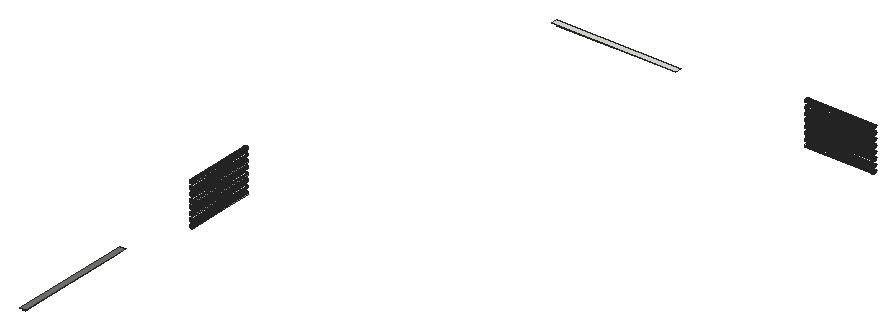
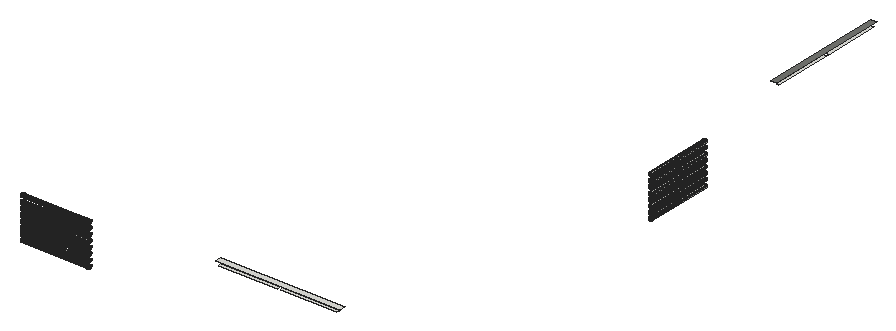
# SketchUp Ruby script. Lengths in inches.
U = 1.inch
M = Sketchup.active_model
def pt(a) = Geom::Point3d.new(a.map { |v| v * U })
def face(e, loops, mat)
  f = e.add_face(loops[0].map { |a| pt(a) })
  loops[1..].each { |l| e.add_face(l.map { |a| pt(a) }).erase! }
  f.material = f.back_material = mat if mat
  f
end
# faces: each face lists its corners as indices into pts; further lists are holes
def faces(e, pts, list, mat = nil) = list.each { |f| face(e, (f[0].is_a?(Array) ? f : [f]).map { |l| l.map { |i| pts[i] } }, mat) }
# xy, xz, yz: faces in a plane at the given z, y or x. An outline is a flat list of corners, or four numbers for a rectangle; further outlines are holes
def ring(l) = l.size == 4 ? [[l[0], l[1]], [l[2], l[1]], [l[2], l[3]], [l[0], l[3]]] : l.each_slice(2).to_a
def flat(e, list, mat, &to3) = list.each { |f| face(e, (f[0].is_a?(Array) ? f : [f]).map { |l| ring(l).map { |u, v| to3.(u, v) } }, mat) }
def xy(e, z, list, mat = nil) = flat(e, list, mat) { |x, y| [x, y, z] }
def xz(e, y, list, mat = nil) = flat(e, list, mat) { |x, z| [x, y, z] }
def yz(e, x, list, mat = nil) = flat(e, list, mat) { |y, z| [x, y, z] }
def lines(e, pts, list) = list.each { |a, b| e.add_line(pt(pts[a]), pt(pts[b])) }
# prism: a flat outline (further loops are holes) pulled along v
def prism(e, loops, v, mat = nil)
  f = face(e, loops, mat); d = Geom::Vector3d.new(v.map { |x| x * U })
  f.pushpull(f.normal.samedirection?(d) ? d.length : -d.length)
end
def box(e, o, s, mat = nil) = prism(e, [[o, [o[0] + s[0], o[1], o[2]], [o[0] + s[0], o[1] + s[1], o[2]], [o[0], o[1] + s[1], o[2]]]], [0, 0, s[2]], mat)
def at(x, y, z, deg = 0) = Geom::Transformation.translation(pt([x, y, z])) * Geom::Transformation.rotation(ORIGIN, Z_AXIS, deg.degrees)
def axes(o, x, y, z) = Geom::Transformation.new([*x, 0, *y, 0, *z, 0, *pt(o).to_a, 1])
def part(name) = M.definitions.add(name)
# library, detail: a bought-in or finely detailed component or shape, given as its bounding box
def library(name, o, s) = part(name).tap { |d| box(d.entities, o, s) }
def detail(e, o, s) = box(e.add_group.entities, o, s)
def put(e, d, t, mat = nil) = e.add_instance(d, t).tap { |i| i.material = mat if mat }
def group(e, t, mat = nil) = e.add_group.tap { |g| g.transformation = t; g.material = mat if mat }.entities
root = M.entities
M.materials.add("[Metal Seamed]").color = [118, 119, 115]
xy(root,1007.61,[[120,175.92,126,293.77],[120,299.77,126,423.61],[211.11,1458.8125,328.96,1464.8125],[334.96,1458.8125,458.8,1464.8125]])
xy(root,1013.61,[[205.11,1452.8125,464.8,1464.8125]])
xy(root,1013.61,[[120,169.92,132,429.61]],"[Metal Seamed]")
p = [[83.53,662.8,933.02],[82.57,662.8,933.14],[82.57,806.17,933.14],[83.53,806.17,933.02],[84.48,662.8,933.14],[84.48,806.17,933.14],
  [697.99,1500.33,933.14],[697.99,1501.28,933.02],[841.36,1501.28,933.02],[841.36,1500.33,933.14],[697.99,1502.24,933.14],[841.36,1502.24,933.14],
  [81.68,662.8,933.51],[81.68,806.17,933.51],[85.37,662.8,933.51],[85.37,806.17,933.51],[697.99,1499.44,933.51],[841.36,1499.44,933.51],
  [697.99,1503.13,933.51],[841.36,1503.13,933.51],[80.92,662.8,934.1],[80.92,806.17,934.1],[86.13,662.8,934.1],[86.13,806.17,934.1],
  [697.99,1498.68,934.1],[841.36,1498.68,934.1],[697.99,1503.89,934.1],[841.36,1503.89,934.1],[80.33,662.8,934.86],[80.33,806.17,934.86],
  [86.72,662.8,934.86],[86.72,806.17,934.86],[697.99,1498.09,934.86],[841.36,1498.09,934.86],[697.99,1504.48,934.86],[841.36,1504.48,934.86],
  [79.97,662.8,935.75],[79.97,806.17,935.75],[87.09,662.8,935.75],[87.09,806.17,935.75],[697.99,1497.72,935.75],[841.36,1497.72,935.75],
  [697.99,1504.85,935.75],[841.36,1504.85,935.75],[79.84,662.8,936.7],[79.84,806.17,936.7],[87.21,662.8,936.7],[87.21,806.17,936.7],
  [697.99,1497.6,936.7],[841.36,1497.6,936.7],[697.99,1504.97,936.7],[841.36,1504.97,936.7],[79.97,662.8,937.66],[79.97,806.17,937.66],
  [87.09,662.8,937.66],[87.09,806.17,937.66],[697.99,1497.72,937.66],[841.36,1497.72,937.66],[697.99,1504.85,937.66],[841.36,1504.85,937.66],
  [80.33,662.8,938.55],[80.33,806.17,938.55],[86.72,662.8,938.55],[86.72,806.17,938.55],[697.99,1498.09,938.55],[841.36,1498.09,938.55],
  [697.99,1504.48,938.55],[841.36,1504.48,938.55],[80.92,662.8,939.3125],[80.92,806.17,939.3125],[86.13,662.8,939.3125],[86.13,806.17,939.3125],
  [697.99,1498.68,939.3125],[841.36,1498.68,939.3125],[697.99,1503.89,939.3125],[841.36,1503.89,939.3125],[81.68,662.8,939.9],[81.68,806.17,939.9],
  [85.37,662.8,939.9],[85.37,806.17,939.9],[697.99,1499.44,939.9],[841.36,1499.44,939.9],[697.99,1503.13,939.9],[841.36,1503.13,939.9],
  [82.57,662.8,940.27],[82.57,806.17,940.27],[84.48,662.8,940.27],[84.48,806.17,940.27],[697.99,1500.33,940.27],[841.36,1500.33,940.27],
  [697.99,1502.24,940.27],[841.36,1502.24,940.27],[83.53,662.8,940.39],[83.53,806.17,940.39],[697.99,1501.28,940.39],[841.36,1501.28,940.39],
  [83.53,662.8,945.02],[82.57,662.8,945.14],[82.57,806.17,945.14],[83.53,806.17,945.02],[84.48,662.8,945.14],[84.48,806.17,945.14],
  [697.99,1500.33,945.14],[697.99,1501.28,945.02],[841.36,1501.28,945.02],[841.36,1500.33,945.14],[697.99,1502.24,945.14],[841.36,1502.24,945.14],
  [81.68,662.8,945.51],[81.68,806.17,945.51],[85.37,662.8,945.51],[85.37,806.17,945.51],[697.99,1499.44,945.51],[841.36,1499.44,945.51],
  [697.99,1503.13,945.51],[841.36,1503.13,945.51],[80.92,662.8,946.1],[80.92,806.17,946.1],[86.13,662.8,946.1],[86.13,806.17,946.1],
  [697.99,1498.68,946.1],[841.36,1498.68,946.1],[697.99,1503.89,946.1],[841.36,1503.89,946.1],[80.33,662.8,946.86],[80.33,806.17,946.86],
  [86.72,662.8,946.86],[86.72,806.17,946.86],[697.99,1498.09,946.86],[841.36,1498.09,946.86],[697.99,1504.48,946.86],[841.36,1504.48,946.86],
  [79.97,662.8,947.75],[79.97,806.17,947.75],[87.09,662.8,947.75],[87.09,806.17,947.75],[697.99,1497.72,947.75],[841.36,1497.72,947.75],
  [697.99,1504.85,947.75],[841.36,1504.85,947.75],[79.84,662.8,948.7],[79.84,806.17,948.7],[87.21,662.8,948.7],[87.21,806.17,948.7],
  [697.99,1497.6,948.7],[841.36,1497.6,948.7],[697.99,1504.97,948.7],[841.36,1504.97,948.7],[79.97,662.8,949.66],[79.97,806.17,949.66],
  [87.09,662.8,949.66],[87.09,806.17,949.66],[697.99,1497.72,949.66],[841.36,1497.72,949.66],[697.99,1504.85,949.66],[841.36,1504.85,949.66],
  [80.33,662.8,950.55],[80.33,806.17,950.55],[86.72,662.8,950.55],[86.72,806.17,950.55],[697.99,1498.09,950.55],[841.36,1498.09,950.55],
  [697.99,1504.48,950.55],[841.36,1504.48,950.55],[80.92,662.8,951.3125],[80.92,806.17,951.3125],[86.13,662.8,951.3125],[86.13,806.17,951.3125],
  [697.99,1498.68,951.3125],[841.36,1498.68,951.3125],[697.99,1503.89,951.3125],[841.36,1503.89,951.3125],[81.68,662.8,951.9],[81.68,806.17,951.9],
  [85.37,662.8,951.9],[85.37,806.17,951.9],[697.99,1499.44,951.9],[841.36,1499.44,951.9],[697.99,1503.13,951.9],[841.36,1503.13,951.9],
  [82.57,662.8,952.27],[82.57,806.17,952.27],[84.48,662.8,952.27],[84.48,806.17,952.27],[697.99,1500.33,952.27],[841.36,1500.33,952.27],
  [697.99,1502.24,952.27],[841.36,1502.24,952.27],[83.53,662.8,952.39],[83.53,806.17,952.39],[697.99,1501.28,952.39],[841.36,1501.28,952.39],
  [83.53,662.8,957.02],[82.57,662.8,957.14],[82.57,806.17,957.14],[83.53,806.17,957.02],[84.48,662.8,957.14],[84.48,806.17,957.14],
  [697.99,1500.33,957.14],[697.99,1501.28,957.02],[841.36,1501.28,957.02],[841.36,1500.33,957.14],[697.99,1502.24,957.14],[841.36,1502.24,957.14],
  [81.68,662.8,957.51],[81.68,806.17,957.51],[85.37,662.8,957.51],[85.37,806.17,957.51],[697.99,1499.44,957.51],[841.36,1499.44,957.51],
  [697.99,1503.13,957.51],[841.36,1503.13,957.51],[80.92,662.8,958.1],[80.92,806.17,958.1],[86.13,662.8,958.1],[86.13,806.17,958.1],
  [697.99,1498.68,958.1],[841.36,1498.68,958.1],[697.99,1503.89,958.1],[841.36,1503.89,958.1],[80.33,662.8,958.86],[80.33,806.17,958.86],
  [86.72,662.8,958.86],[86.72,806.17,958.86],[697.99,1498.09,958.86],[841.36,1498.09,958.86],[697.99,1504.48,958.86],[841.36,1504.48,958.86],
  [79.97,662.8,959.75],[79.97,806.17,959.75],[87.09,662.8,959.75],[87.09,806.17,959.75],[697.99,1497.72,959.75],[841.36,1497.72,959.75],
  [697.99,1504.85,959.75],[841.36,1504.85,959.75],[79.84,662.8,960.7],[79.84,806.17,960.7],[87.21,662.8,960.7],[87.21,806.17,960.7],
  [697.99,1497.6,960.7],[841.36,1497.6,960.7],[697.99,1504.97,960.7],[841.36,1504.97,960.7],[79.97,662.8,961.66],[79.97,806.17,961.66],
  [87.09,662.8,961.66],[87.09,806.17,961.66],[697.99,1497.72,961.66],[841.36,1497.72,961.66],[697.99,1504.85,961.66],[841.36,1504.85,961.66],
  [80.33,662.8,962.55],[80.33,806.17,962.55],[86.72,662.8,962.55],[86.72,806.17,962.55],[697.99,1498.09,962.55],[841.36,1498.09,962.55],
  [697.99,1504.48,962.55],[841.36,1504.48,962.55],[80.92,662.8,963.3125],[80.92,806.17,963.3125],[86.13,662.8,963.3125],[86.13,806.17,963.3125],
  [697.99,1498.68,963.3125],[841.36,1498.68,963.3125],[697.99,1503.89,963.3125],[841.36,1503.89,963.3125],[81.68,662.8,963.9],[81.68,806.17,963.9],
  [85.37,662.8,963.9],[85.37,806.17,963.9],[697.99,1499.44,963.9],[841.36,1499.44,963.9],[697.99,1503.13,963.9],[841.36,1503.13,963.9],
  [82.57,662.8,964.27],[82.57,806.17,964.27],[84.48,662.8,964.27],[84.48,806.17,964.27],[697.99,1500.33,964.27],[841.36,1500.33,964.27],
  [697.99,1502.24,964.27],[841.36,1502.24,964.27],[83.53,662.8,964.39],[83.53,806.17,964.39],[697.99,1501.28,964.39],[841.36,1501.28,964.39],
  [83.53,662.8,969.02],[82.57,662.8,969.14],[82.57,806.17,969.14],[83.53,806.17,969.02],[84.48,662.8,969.14],[84.48,806.17,969.14],
  [697.99,1500.33,969.14],[697.99,1501.28,969.02],[841.36,1501.28,969.02],[841.36,1500.33,969.14],[697.99,1502.24,969.14],[841.36,1502.24,969.14],
  [81.68,662.8,969.51],[81.68,806.17,969.51],[85.37,662.8,969.51],[85.37,806.17,969.51],[697.99,1499.44,969.51],[841.36,1499.44,969.51],
  [697.99,1503.13,969.51],[841.36,1503.13,969.51],[80.92,662.8,970.1],[80.92,806.17,970.1],[86.13,662.8,970.1],[86.13,806.17,970.1],
  [697.99,1498.68,970.1],[841.36,1498.68,970.1],[697.99,1503.89,970.1],[841.36,1503.89,970.1],[80.33,662.8,970.86],[80.33,806.17,970.86],
  [86.72,662.8,970.86],[86.72,806.17,970.86],[697.99,1498.09,970.86],[841.36,1498.09,970.86],[697.99,1504.48,970.86],[841.36,1504.48,970.86],
  [79.97,662.8,971.75],[79.97,806.17,971.75],[87.09,662.8,971.75],[87.09,806.17,971.75],[697.99,1497.72,971.75],[841.36,1497.72,971.75],
  [697.99,1504.85,971.75],[841.36,1504.85,971.75],[79.84,662.8,972.7],[79.84,806.17,972.7],[87.21,662.8,972.7],[87.21,806.17,972.7],
  [697.99,1497.6,972.7],[841.36,1497.6,972.7],[697.99,1504.97,972.7],[841.36,1504.97,972.7],[79.97,662.8,973.66],[79.97,806.17,973.66],
  [87.09,662.8,973.66],[87.09,806.17,973.66],[697.99,1497.72,973.66],[841.36,1497.72,973.66],[697.99,1504.85,973.66],[841.36,1504.85,973.66],
  [80.33,662.8,974.55],[80.33,806.17,974.55],[86.72,662.8,974.55],[86.72,806.17,974.55],[697.99,1498.09,974.55],[841.36,1498.09,974.55],
  [697.99,1504.48,974.55],[841.36,1504.48,974.55],[80.92,662.8,975.3125],[80.92,806.17,975.3125],[86.13,662.8,975.3125],[86.13,806.17,975.3125],
  [697.99,1498.68,975.3125],[841.36,1498.68,975.3125],[697.99,1503.89,975.3125],[841.36,1503.89,975.3125],[81.68,662.8,975.9],[81.68,806.17,975.9],
  [85.37,662.8,975.9],[85.37,806.17,975.9],[697.99,1499.44,975.9],[841.36,1499.44,975.9],[697.99,1503.13,975.9],[841.36,1503.13,975.9],
  [82.57,662.8,976.27],[82.57,806.17,976.27],[84.48,662.8,976.27],[84.48,806.17,976.27],[697.99,1500.33,976.27],[841.36,1500.33,976.27],
  [697.99,1502.24,976.27],[841.36,1502.24,976.27],[83.53,662.8,976.39],[83.53,806.17,976.39],[697.99,1501.28,976.39],[841.36,1501.28,976.39],
  [83.53,662.8,981.02],[82.57,662.8,981.14],[82.57,806.17,981.14],[83.53,806.17,981.02],[84.48,662.8,981.14],[84.48,806.17,981.14],
  [697.99,1500.33,981.14],[697.99,1501.28,981.02],[841.36,1501.28,981.02],[841.36,1500.33,981.14],[697.99,1502.24,981.14],[841.36,1502.24,981.14],
  [81.68,662.8,981.51],[81.68,806.17,981.51],[85.37,662.8,981.51],[85.37,806.17,981.51],[697.99,1499.44,981.51],[841.36,1499.44,981.51],
  [697.99,1503.13,981.51],[841.36,1503.13,981.51],[80.92,662.8,982.1],[80.92,806.17,982.1],[86.13,662.8,982.1],[86.13,806.17,982.1],
  [697.99,1498.68,982.1],[841.36,1498.68,982.1],[697.99,1503.89,982.1],[841.36,1503.89,982.1],[80.33,662.8,982.86],[80.33,806.17,982.86],
  [86.72,662.8,982.86],[86.72,806.17,982.86],[697.99,1498.09,982.86],[841.36,1498.09,982.86],[697.99,1504.48,982.86],[841.36,1504.48,982.86],
  [79.97,662.8,983.75],[79.97,806.17,983.75],[87.09,662.8,983.75],[87.09,806.17,983.75],[697.99,1497.72,983.75],[841.36,1497.72,983.75],
  [697.99,1504.85,983.75],[841.36,1504.85,983.75],[79.84,662.8,984.7],[79.84,806.17,984.7],[87.21,662.8,984.7],[87.21,806.17,984.7],
  [697.99,1497.6,984.7],[841.36,1497.6,984.7],[697.99,1504.97,984.7],[841.36,1504.97,984.7],[79.97,662.8,985.66],[79.97,806.17,985.66],
  [87.09,662.8,985.66],[87.09,806.17,985.66],[697.99,1497.72,985.66],[841.36,1497.72,985.66],[697.99,1504.85,985.66],[841.36,1504.85,985.66],
  [80.33,662.8,986.55],[80.33,806.17,986.55],[86.72,662.8,986.55],[86.72,806.17,986.55],[697.99,1498.09,986.55],[841.36,1498.09,986.55],
  [697.99,1504.48,986.55],[841.36,1504.48,986.55],[80.92,662.8,987.3125],[80.92,806.17,987.3125],[86.13,662.8,987.3125],[86.13,806.17,987.3125],
  [697.99,1498.68,987.3125],[841.36,1498.68,987.3125],[697.99,1503.89,987.3125],[841.36,1503.89,987.3125],[81.68,662.8,987.9],[81.68,806.17,987.9],
  [85.37,662.8,987.9],[85.37,806.17,987.9],[697.99,1499.44,987.9],[841.36,1499.44,987.9],[697.99,1503.13,987.9],[841.36,1503.13,987.9],
  [82.57,662.8,988.27],[82.57,806.17,988.27],[84.48,662.8,988.27],[84.48,806.17,988.27],[697.99,1500.33,988.27],[841.36,1500.33,988.27],
  [697.99,1502.24,988.27],[841.36,1502.24,988.27],[83.53,662.8,988.39],[83.53,806.17,988.39],[697.99,1501.28,988.39],[841.36,1501.28,988.39],
  [83.53,662.8,993.02],[82.57,662.8,993.14],[82.57,806.17,993.14],[83.53,806.17,993.02],[84.48,662.8,993.14],[84.48,806.17,993.14],
  [697.99,1500.33,993.14],[697.99,1501.28,993.02],[841.36,1501.28,993.02],[841.36,1500.33,993.14],[697.99,1502.24,993.14],[841.36,1502.24,993.14],
  [81.68,662.8,993.51],[81.68,806.17,993.51],[85.37,662.8,993.51],[85.37,806.17,993.51],[697.99,1499.44,993.51],[841.36,1499.44,993.51],
  [697.99,1503.13,993.51],[841.36,1503.13,993.51],[80.92,662.8,994.1],[80.92,806.17,994.1],[86.13,662.8,994.1],[86.13,806.17,994.1],
  [697.99,1498.68,994.1],[841.36,1498.68,994.1],[697.99,1503.89,994.1],[841.36,1503.89,994.1],[80.33,662.8,994.86],[80.33,806.17,994.86],
  [86.72,662.8,994.86],[86.72,806.17,994.86],[697.99,1498.09,994.86],[841.36,1498.09,994.86],[697.99,1504.48,994.86],[841.36,1504.48,994.86],
  [79.97,662.8,995.75],[79.97,806.17,995.75],[87.09,662.8,995.75],[87.09,806.17,995.75],[697.99,1497.72,995.75],[841.36,1497.72,995.75],
  [697.99,1504.85,995.75],[841.36,1504.85,995.75],[79.84,662.8,996.7],[79.84,806.17,996.7],[87.21,662.8,996.7],[87.21,806.17,996.7],
  [697.99,1497.6,996.7],[841.36,1497.6,996.7],[697.99,1504.97,996.7],[841.36,1504.97,996.7],[79.97,662.8,997.66],[79.97,806.17,997.66],
  [87.09,662.8,997.66],[87.09,806.17,997.66],[697.99,1497.72,997.66],[841.36,1497.72,997.66],[697.99,1504.85,997.66],[841.36,1504.85,997.66],
  [80.33,662.8,998.55],[80.33,806.17,998.55],[86.72,662.8,998.55],[86.72,806.17,998.55],[697.99,1498.09,998.55],[841.36,1498.09,998.55],
  [697.99,1504.48,998.55],[841.36,1504.48,998.55],[80.92,662.8,999.3125],[80.92,806.17,999.3125],[86.13,662.8,999.3125],[86.13,806.17,999.3125],
  [697.99,1498.68,999.3125],[841.36,1498.68,999.3125],[697.99,1503.89,999.3125],[841.36,1503.89,999.3125],[81.68,662.8,999.9],[81.68,806.17,999.9],
  [85.37,662.8,999.9],[85.37,806.17,999.9],[697.99,1499.44,999.9],[841.36,1499.44,999.9],[697.99,1503.13,999.9],[841.36,1503.13,999.9],
  [82.57,662.8,1000.27],[82.57,806.17,1000.27],[84.48,662.8,1000.27],[84.48,806.17,1000.27],[697.99,1500.33,1000.27],[841.36,1500.33,1000.27],
  [697.99,1502.24,1000.27],[841.36,1502.24,1000.27],[83.53,662.8,1000.39],[83.53,806.17,1000.39],[697.99,1501.28,1000.39],[841.36,1501.28,1000.39],
  [83.53,662.8,1005.02],[82.57,662.8,1005.14],[82.57,806.17,1005.14],[83.53,806.17,1005.02],[84.48,662.8,1005.14],[84.48,806.17,1005.14],
  [697.99,1500.33,1005.14],[697.99,1501.28,1005.02],[841.36,1501.28,1005.02],[841.36,1500.33,1005.14],[697.99,1502.24,1005.14],[841.36,1502.24,1005.14],
  [81.68,662.8,1005.51],[81.68,806.17,1005.51],[85.37,662.8,1005.51],[85.37,806.17,1005.51],[697.99,1499.44,1005.51],[841.36,1499.44,1005.51],
  [697.99,1503.13,1005.51],[841.36,1503.13,1005.51],[80.92,662.8,1006.1],[80.92,806.17,1006.1],[86.13,662.8,1006.1],[86.13,806.17,1006.1],
  [697.99,1498.68,1006.1],[841.36,1498.68,1006.1],[697.99,1503.89,1006.1],[841.36,1503.89,1006.1],[80.33,662.8,1006.86],[80.33,806.17,1006.86],
  [86.72,662.8,1006.86],[86.72,806.17,1006.86],[697.99,1498.09,1006.86],[841.36,1498.09,1006.86],[697.99,1504.48,1006.86],[841.36,1504.48,1006.86],
  [79.97,662.8,1007.75],[79.97,806.17,1007.75],[87.09,662.8,1007.75],[87.09,806.17,1007.75],[697.99,1497.72,1007.75],[841.36,1497.72,1007.75],
  [697.99,1504.85,1007.75],[841.36,1504.85,1007.75],[79.84,662.8,1008.7],[79.84,806.17,1008.7],[87.21,662.8,1008.7],[87.21,806.17,1008.7],
  [697.99,1497.6,1008.7],[841.36,1497.6,1008.7],[697.99,1504.97,1008.7],[841.36,1504.97,1008.7],[79.97,662.8,1009.66],[79.97,806.17,1009.66],
  [87.09,662.8,1009.66],[87.09,806.17,1009.66],[697.99,1497.72,1009.66],[841.36,1497.72,1009.66],[697.99,1504.85,1009.66],[841.36,1504.85,1009.66],
  [80.33,662.8,1010.55],[80.33,806.17,1010.55],[86.72,662.8,1010.55],[86.72,806.17,1010.55],[697.99,1498.09,1010.55],[841.36,1498.09,1010.55],
  [697.99,1504.48,1010.55],[841.36,1504.48,1010.55],[80.92,662.8,1011.3125],[80.92,806.17,1011.3125],[86.13,662.8,1011.3125],[86.13,806.17,1011.3125],
  [697.99,1498.68,1011.3125],[841.36,1498.68,1011.3125],[697.99,1503.89,1011.3125],[841.36,1503.89,1011.3125],[81.68,662.8,1011.9],[81.68,806.17,1011.9],
  [85.37,662.8,1011.9],[85.37,806.17,1011.9],[697.99,1499.44,1011.9],[841.36,1499.44,1011.9],[697.99,1503.13,1011.9],[841.36,1503.13,1011.9],
  [82.57,662.8,1012.27],[82.57,806.17,1012.27],[84.48,662.8,1012.27],[84.48,806.17,1012.27],[697.99,1500.33,1012.27],[841.36,1500.33,1012.27],
  [697.99,1502.24,1012.27],[841.36,1502.24,1012.27],[83.53,662.8,1012.39],[83.53,806.17,1012.39],[697.99,1501.28,1012.39],[841.36,1501.28,1012.39],
  [83.53,662.8,1017.02],[82.57,662.8,1017.14],[82.57,806.17,1017.14],[83.53,806.17,1017.02],[84.48,662.8,1017.14],[84.48,806.17,1017.14],
  [697.99,1500.33,1017.14],[697.99,1501.28,1017.02],[841.36,1501.28,1017.02],[841.36,1500.33,1017.14],[697.99,1502.24,1017.14],[841.36,1502.24,1017.14],
  [81.68,662.8,1017.51],[81.68,806.17,1017.51],[85.37,662.8,1017.51],[85.37,806.17,1017.51],[697.99,1499.44,1017.51],[841.36,1499.44,1017.51],
  [697.99,1503.13,1017.51],[841.36,1503.13,1017.51],[80.92,662.8,1018.1],[80.92,806.17,1018.1],[86.13,662.8,1018.1],[86.13,806.17,1018.1],
  [697.99,1498.68,1018.1],[841.36,1498.68,1018.1],[697.99,1503.89,1018.1],[841.36,1503.89,1018.1],[80.33,662.8,1018.86],[80.33,806.17,1018.86],
  [86.72,662.8,1018.86],[86.72,806.17,1018.86],[697.99,1498.09,1018.86],[841.36,1498.09,1018.86],[697.99,1504.48,1018.86],[841.36,1504.48,1018.86],
  [79.97,662.8,1019.75],[79.97,806.17,1019.75],[87.09,662.8,1019.75],[87.09,806.17,1019.75],[697.99,1497.72,1019.75],[841.36,1497.72,1019.75],
  [697.99,1504.85,1019.75],[841.36,1504.85,1019.75],[79.84,662.8,1020.7],[79.84,806.17,1020.7],[87.21,662.8,1020.7],[87.21,806.17,1020.7],
  [697.99,1497.6,1020.7],[841.36,1497.6,1020.7],[697.99,1504.97,1020.7],[841.36,1504.97,1020.7],[79.97,662.8,1021.66],[79.97,806.17,1021.66],
  [87.09,662.8,1021.66],[87.09,806.17,1021.66],[697.99,1497.72,1021.66],[841.36,1497.72,1021.66],[697.99,1504.85,1021.66],[841.36,1504.85,1021.66],
  [80.33,662.8,1022.55],[80.33,806.17,1022.55],[86.72,662.8,1022.55],[86.72,806.17,1022.55],[697.99,1498.09,1022.55],[841.36,1498.09,1022.55],
  [697.99,1504.48,1022.55],[841.36,1504.48,1022.55],[80.92,662.8,1023.3125],[80.92,806.17,1023.3125],[86.13,662.8,1023.3125],[86.13,806.17,1023.3125],
  [697.99,1498.68,1023.3125],[841.36,1498.68,1023.3125],[697.99,1503.89,1023.3125],[841.36,1503.89,1023.3125],[81.68,662.8,1023.9],[81.68,806.17,1023.9],
  [85.37,662.8,1023.9],[85.37,806.17,1023.9],[697.99,1499.44,1023.9],[841.36,1499.44,1023.9],[697.99,1503.13,1023.9],[841.36,1503.13,1023.9],
  [82.57,662.8,1024.27],[82.57,806.17,1024.27],[84.48,662.8,1024.27],[84.48,806.17,1024.27],[697.99,1500.33,1024.27],[841.36,1500.33,1024.27],
  [697.99,1502.24,1024.27],[841.36,1502.24,1024.27],[83.53,662.8,1024.39],[83.53,806.17,1024.39],[697.99,1501.28,1024.39],[841.36,1501.28,1024.39]]
faces(root,p,[[0,1,2,3],[4,0,3,5],[6,7,8,9],[7,10,11,8],[1,12,13,2],[14,4,5,15],[16,6,9,17],[10,18,19,11],
  [12,20,21,13],[22,14,15,23],[24,16,17,25],[18,26,27,19],[20,28,29,21],[30,22,23,31],[32,24,25,33],[26,34,35,27],
  [28,36,37,29],[38,30,31,39],[40,32,33,41],[34,42,43,35],[36,44,45,37],[46,38,39,47],[48,40,41,49],[42,50,51,43],
  [44,52,53,45],[54,46,47,55],[56,48,49,57],[50,58,59,51],[52,60,61,53],[62,54,55,63],[64,56,57,65],[58,66,67,59],
  [60,68,69,61],[70,62,63,71],[72,64,65,73],[66,74,75,67],[68,76,77,69],[78,70,71,79],[80,72,73,81],[74,82,83,75],
  [76,84,85,77],[86,78,79,87],[88,80,81,89],[82,90,91,83],[84,92,93,85],[92,86,87,93],[94,88,89,95],[90,94,95,91],
  [96,97,98,99],[100,96,99,101],[102,103,104,105],[103,106,107,104],[97,108,109,98],[110,100,101,111],[112,102,105,113],[106,114,115,107],
  [108,116,117,109],[118,110,111,119],[120,112,113,121],[114,122,123,115],[116,124,125,117],[126,118,119,127],[128,120,121,129],[122,130,131,123],
  [124,132,133,125],[134,126,127,135],[136,128,129,137],[130,138,139,131],[132,140,141,133],[142,134,135,143],[144,136,137,145],[138,146,147,139],
  [140,148,149,141],[150,142,143,151],[152,144,145,153],[146,154,155,147],[148,156,157,149],[158,150,151,159],[160,152,153,161],[154,162,163,155],
  [156,164,165,157],[166,158,159,167],[168,160,161,169],[162,170,171,163],[164,172,173,165],[174,166,167,175],[176,168,169,177],[170,178,179,171],
  [172,180,181,173],[182,174,175,183],[184,176,177,185],[178,186,187,179],[180,188,189,181],[188,182,183,189],[190,184,185,191],[186,190,191,187],
  [192,193,194,195],[196,192,195,197],[198,199,200,201],[199,202,203,200],[193,204,205,194],[206,196,197,207],[208,198,201,209],[202,210,211,203],
  [204,212,213,205],[214,206,207,215],[216,208,209,217],[210,218,219,211],[212,220,221,213],[222,214,215,223],[224,216,217,225],[218,226,227,219],
  [220,228,229,221],[230,222,223,231],[232,224,225,233],[226,234,235,227],[228,236,237,229],[238,230,231,239],[240,232,233,241],[234,242,243,235],
  [236,244,245,237],[246,238,239,247],[248,240,241,249],[242,250,251,243],[244,252,253,245],[254,246,247,255],[256,248,249,257],[250,258,259,251],
  [252,260,261,253],[262,254,255,263],[264,256,257,265],[258,266,267,259],[260,268,269,261],[270,262,263,271],[272,264,265,273],[266,274,275,267],
  [268,276,277,269],[278,270,271,279],[280,272,273,281],[274,282,283,275],[276,284,285,277],[284,278,279,285],[286,280,281,287],[282,286,287,283],
  [288,289,290,291],[292,288,291,293],[294,295,296,297],[295,298,299,296],[289,300,301,290],[302,292,293,303],[304,294,297,305],[298,306,307,299],
  [300,308,309,301],[310,302,303,311],[312,304,305,313],[306,314,315,307],[308,316,317,309],[318,310,311,319],[320,312,313,321],[314,322,323,315],
  [316,324,325,317],[326,318,319,327],[328,320,321,329],[322,330,331,323],[324,332,333,325],[334,326,327,335],[336,328,329,337],[330,338,339,331],
  [332,340,341,333],[342,334,335,343],[344,336,337,345],[338,346,347,339],[340,348,349,341],[350,342,343,351],[352,344,345,353],[346,354,355,347],
  [348,356,357,349],[358,350,351,359],[360,352,353,361],[354,362,363,355],[356,364,365,357],[366,358,359,367],[368,360,361,369],[362,370,371,363],
  [364,372,373,365],[374,366,367,375],[376,368,369,377],[370,378,379,371],[372,380,381,373],[380,374,375,381],[382,376,377,383],[378,382,383,379],
  [384,385,386,387],[388,384,387,389],[390,391,392,393],[391,394,395,392],[385,396,397,386],[398,388,389,399],[400,390,393,401],[394,402,403,395],
  [396,404,405,397],[406,398,399,407],[408,400,401,409],[402,410,411,403],[404,412,413,405],[414,406,407,415],[416,408,409,417],[410,418,419,411],
  [412,420,421,413],[422,414,415,423],[424,416,417,425],[418,426,427,419],[420,428,429,421],[430,422,423,431],[432,424,425,433],[426,434,435,427],
  [428,436,437,429],[438,430,431,439],[440,432,433,441],[434,442,443,435],[436,444,445,437],[446,438,439,447],[448,440,441,449],[442,450,451,443],
  [444,452,453,445],[454,446,447,455],[456,448,449,457],[450,458,459,451],[452,460,461,453],[462,454,455,463],[464,456,457,465],[458,466,467,459],
  [460,468,469,461],[470,462,463,471],[472,464,465,473],[466,474,475,467],[468,476,477,469],[476,470,471,477],[478,472,473,479],[474,478,479,475],
  [480,481,482,483],[484,480,483,485],[486,487,488,489],[487,490,491,488],[481,492,493,482],[494,484,485,495],[496,486,489,497],[490,498,499,491],
  [492,500,501,493],[502,494,495,503],[504,496,497,505],[498,506,507,499],[500,508,509,501],[510,502,503,511],[512,504,505,513],[506,514,515,507],
  [508,516,517,509],[518,510,511,519],[520,512,513,521],[514,522,523,515],[516,524,525,517],[526,518,519,527],[528,520,521,529],[522,530,531,523],
  [524,532,533,525],[534,526,527,535],[536,528,529,537],[530,538,539,531],[532,540,541,533],[542,534,535,543],[544,536,537,545],[538,546,547,539],
  [540,548,549,541],[550,542,543,551],[552,544,545,553],[546,554,555,547],[548,556,557,549],[558,550,551,559],[560,552,553,561],[554,562,563,555],
  [556,564,565,557],[566,558,559,567],[568,560,561,569],[562,570,571,563],[564,572,573,565],[572,566,567,573],[574,568,569,575],[570,574,575,571],
  [576,577,578,579],[580,576,579,581],[582,583,584,585],[583,586,587,584],[577,588,589,578],[590,580,581,591],[592,582,585,593],[586,594,595,587],
  [588,596,597,589],[598,590,591,599],[600,592,593,601],[594,602,603,595],[596,604,605,597],[606,598,599,607],[608,600,601,609],[602,610,611,603],
  [604,612,613,605],[614,606,607,615],[616,608,609,617],[610,618,619,611],[612,620,621,613],[622,614,615,623],[624,616,617,625],[618,626,627,619],
  [620,628,629,621],[630,622,623,631],[632,624,625,633],[626,634,635,627],[628,636,637,629],[638,630,631,639],[640,632,633,641],[634,642,643,635],
  [636,644,645,637],[646,638,639,647],[648,640,641,649],[642,650,651,643],[644,652,653,645],[654,646,647,655],[656,648,649,657],[650,658,659,651],
  [652,660,661,653],[662,654,655,663],[664,656,657,665],[658,666,667,659],[660,668,669,661],[668,662,663,669],[670,664,665,671],[666,670,671,667],
  [672,673,674,675],[676,672,675,677],[678,679,680,681],[679,682,683,680],[673,684,685,674],[686,676,677,687],[688,678,681,689],[682,690,691,683],
  [684,692,693,685],[694,686,687,695],[696,688,689,697],[690,698,699,691],[692,700,701,693],[702,694,695,703],[704,696,697,705],[698,706,707,699],
  [700,708,709,701],[710,702,703,711],[712,704,705,713],[706,714,715,707],[708,716,717,709],[718,710,711,719],[720,712,713,721],[714,722,723,715],
  [716,724,725,717],[726,718,719,727],[728,720,721,729],[722,730,731,723],[724,732,733,725],[734,726,727,735],[736,728,729,737],[730,738,739,731],
  [732,740,741,733],[742,734,735,743],[744,736,737,745],[738,746,747,739],[740,748,749,741],[750,742,743,751],[752,744,745,753],[746,754,755,747],
  [748,756,757,749],[758,750,751,759],[760,752,753,761],[754,762,763,755],[756,764,765,757],[764,758,759,765],[766,760,761,767],[762,766,767,763]])
